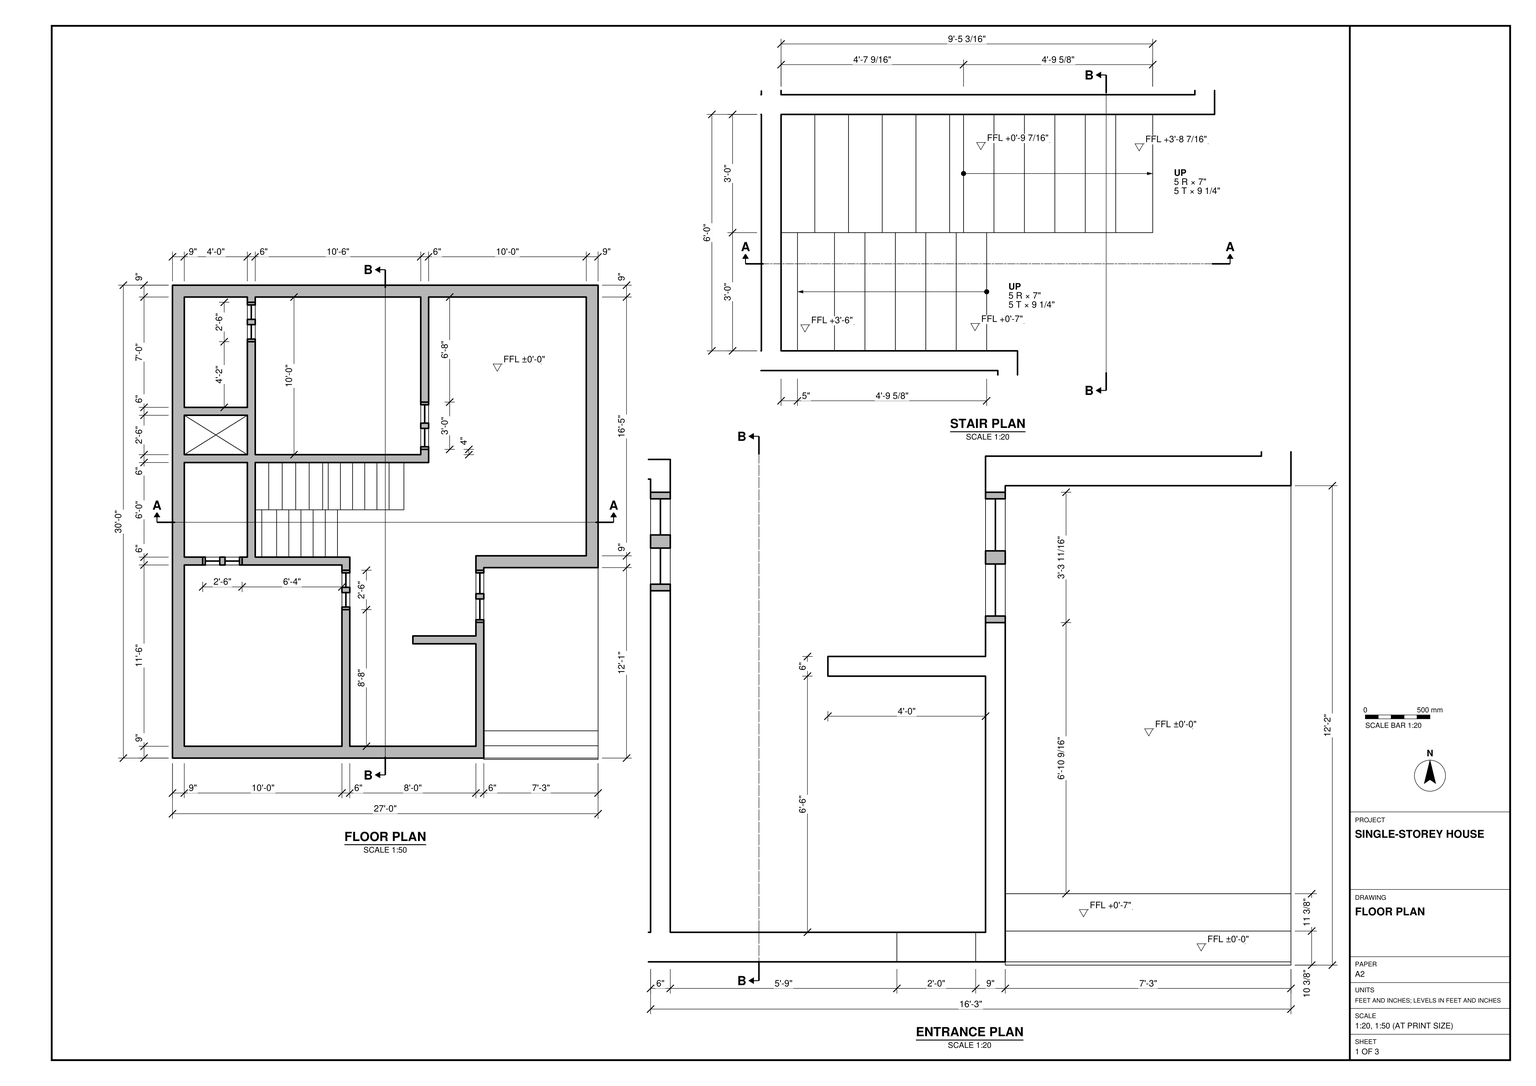
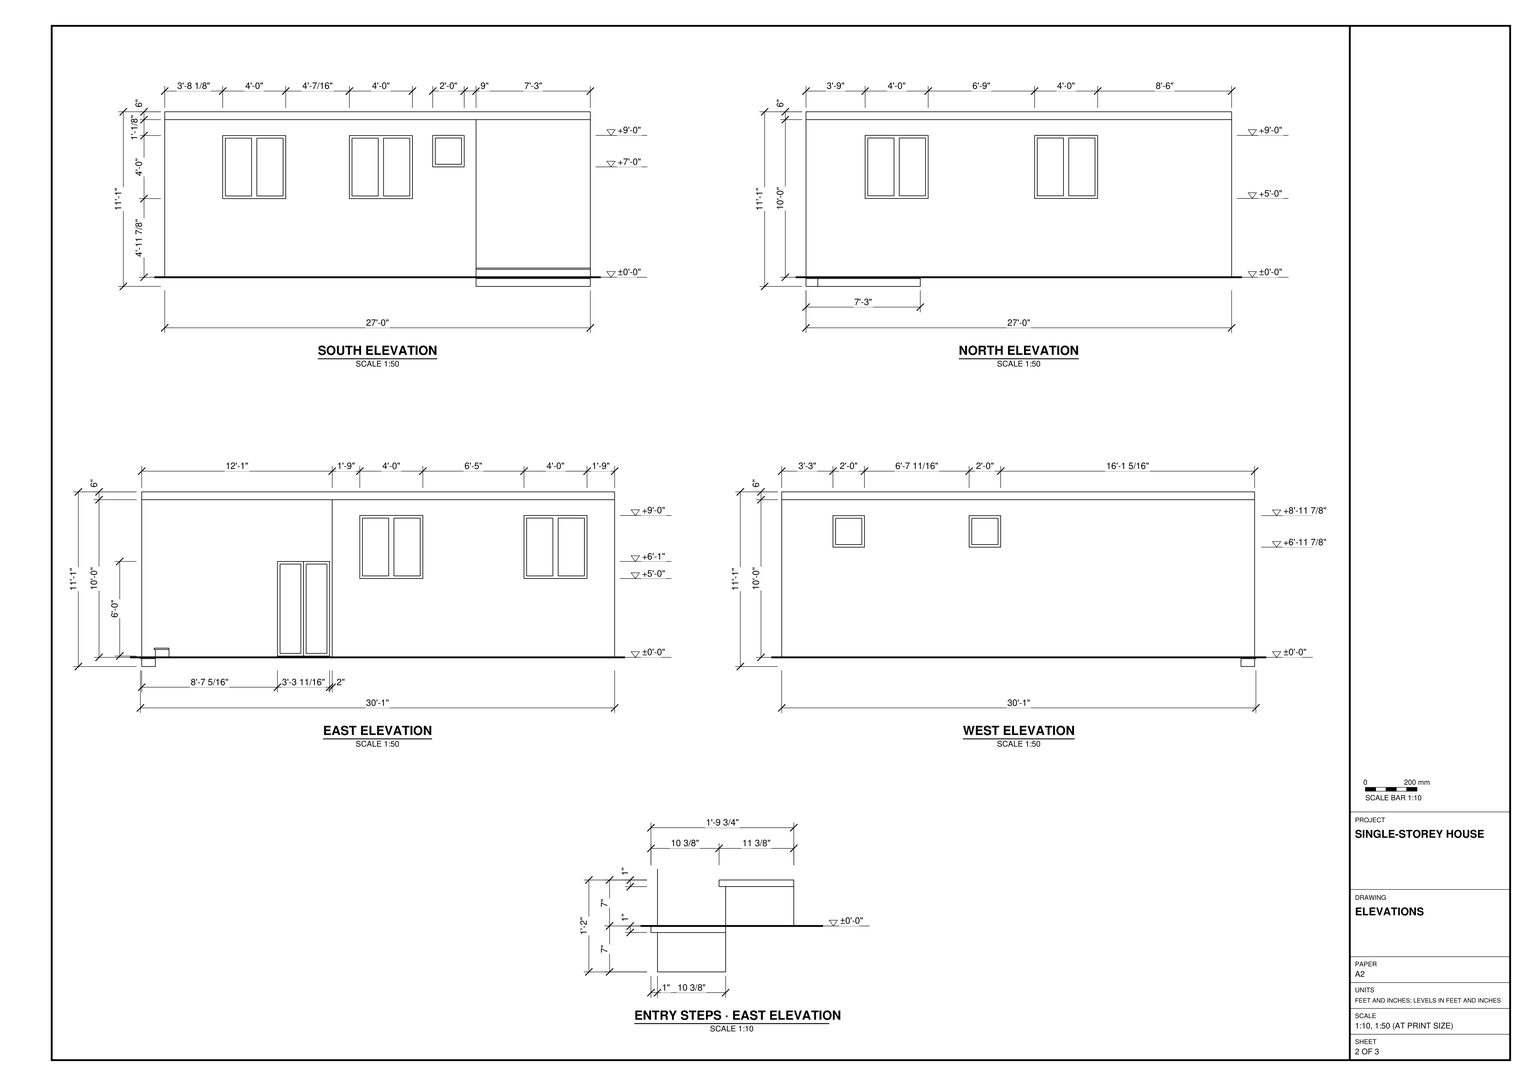
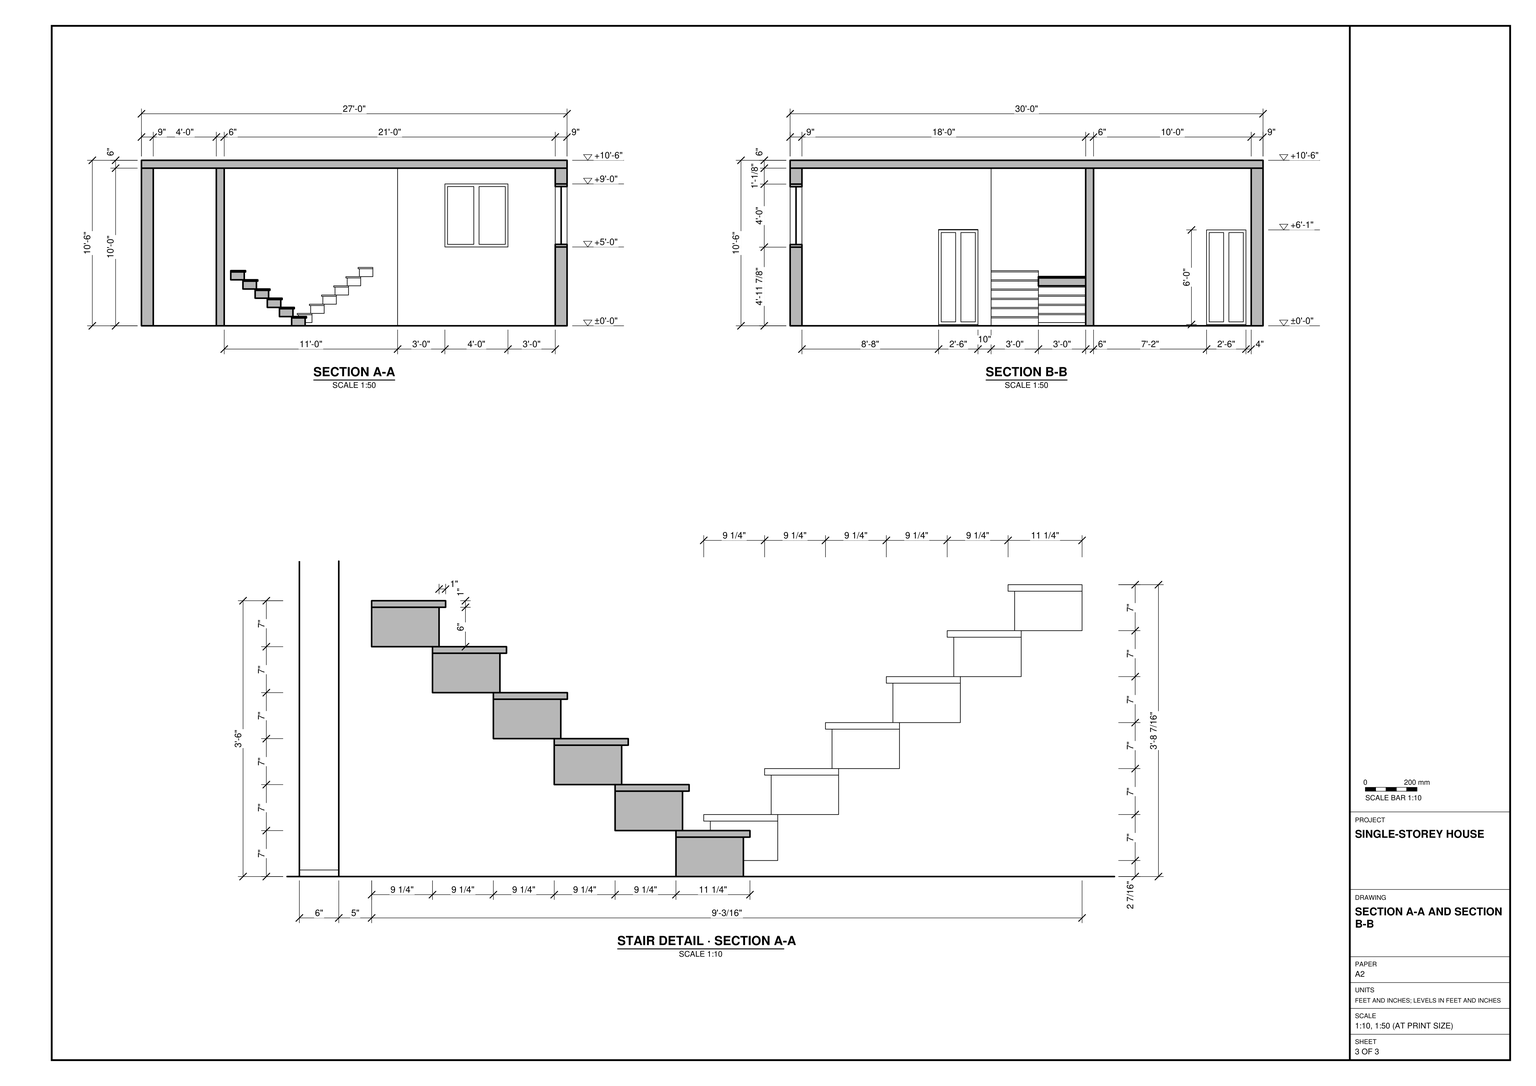
Build the house in SketchUp from task_files/diagram_01.pdf. Work in feet and inches, with the ground-floor finished level at ±0'-0". The overall dimensions are 27'-0" east to west, 30'-1" north to south and 11'-1" from the lowest part of the entry steps to the top of the roof.

Use the floor plan to set out the shell, including the recessed southeast entrance, the narrow rooms along the west side and the partitions around the central stair. Follow the drawn wall thicknesses, distinguishing the 9" exterior walls from the 6" partitions and returns where indicated. Model the floor and flat roof slab. Use the elevations to place the door and window openings and to distinguish the paired panes from the smaller square windows. Use the sections to set the window heights and the underside of the roof.

Model the entrance steps across the width of the recess. For the interior stair, use the stair plan for the position and direction of each flight and the enlarged section for the rises, tread spacing and projecting nosings. Decor and loose items, if used, may be any suitable library components. Keep walls, slabs, roof and any furniture or joinery pieces in separate groups or components, and use components for repeated parts. Save one SketchUp model as output_files/single_storey_house_with_recessed_entrance.skp.

# SketchUp Ruby script. Lengths in inches.
U = 1.inch
M = Sketchup.active_model
def pt(a) = Geom::Point3d.new(a.map { |v| v * U })
def face(e, loops, mat)
  f = e.add_face(loops[0].map { |a| pt(a) })
  loops[1..].each { |l| e.add_face(l.map { |a| pt(a) }).erase! }
  f.material = f.back_material = mat if mat
  f
end
# faces: each face lists its corners as indices into pts; further lists are holes
def faces(e, pts, list, mat = nil) = list.each { |f| face(e, (f[0].is_a?(Array) ? f : [f]).map { |l| l.map { |i| pts[i] } }, mat) }
# xy, xz, yz: faces in a plane at the given z, y or x. An outline is a flat list of corners, or four numbers for a rectangle; further outlines are holes
def ring(l) = l.size == 4 ? [[l[0], l[1]], [l[2], l[1]], [l[2], l[3]], [l[0], l[3]]] : l.each_slice(2).to_a
def flat(e, list, mat, &to3) = list.each { |f| face(e, (f[0].is_a?(Array) ? f : [f]).map { |l| ring(l).map { |u, v| to3.(u, v) } }, mat) }
def xy(e, z, list, mat = nil) = flat(e, list, mat) { |x, y| [x, y, z] }
def xz(e, y, list, mat = nil) = flat(e, list, mat) { |x, z| [x, y, z] }
def yz(e, x, list, mat = nil) = flat(e, list, mat) { |y, z| [x, y, z] }
def lines(e, pts, list) = list.each { |a, b| e.add_line(pt(pts[a]), pt(pts[b])) }
# prism: a flat outline (further loops are holes) pulled along v
def prism(e, loops, v, mat = nil)
  f = face(e, loops, mat); d = Geom::Vector3d.new(v.map { |x| x * U })
  f.pushpull(f.normal.samedirection?(d) ? d.length : -d.length)
end
def box(e, o, s, mat = nil) = prism(e, [[o, [o[0] + s[0], o[1], o[2]], [o[0] + s[0], o[1] + s[1], o[2]], [o[0], o[1] + s[1], o[2]]]], [0, 0, s[2]], mat)
def at(x, y, z, deg = 0) = Geom::Transformation.translation(pt([x, y, z])) * Geom::Transformation.rotation(ORIGIN, Z_AXIS, deg.degrees)
def axes(o, x, y, z) = Geom::Transformation.new([*x, 0, *y, 0, *z, 0, *pt(o).to_a, 1])
def part(name) = M.definitions.add(name)
# library, detail: a bought-in or finely detailed component or shape, given as its bounding box
def library(name, o, s) = part(name).tap { |d| box(d.entities, o, s) }
def detail(e, o, s) = box(e.add_group.entities, o, s)
def put(e, d, t, mat = nil) = e.add_instance(d, t).tap { |i| i.material = mat if mat }
def group(e, t, mat = nil) = e.add_group.tap { |g| g.transformation = t; g.material = mat if mat }.entities
root = M.entities
M.materials.add("[Checker Plate]").color = [245, 245, 245]
M.materials.add("[Granite Tile]").color = [155, 148, 143]
M.materials.add("[Tile Travertine 2 inch]").color = [181, 178, 172]
M.materials.add("[Translucent Glass Blue]").color = [100, 149, 237]
M.materials["[Translucent Glass Blue]"].alpha = 0.5
M.materials.add("[Translucent Glass Corrugated]").color = [141, 158, 145]
M.materials["[Translucent Glass Corrugated]"].alpha = 0.8
M.materials.add("[Wood Bamboo]").color = [177, 105, 43]
M.materials.add("[Wood Cherry Original]").color = [152, 86, 42]
M.materials.add("[Wood Veneer 02]").color = [190, 128, 91]
c1 = part("Group\#5")
xy(c1.entities,0,[[0,0,9,24],[0,24,9,48]])
xy(c1.entities,2,[[0,2,4.5,22],[4.5,2,9,22],[0,26,4.5,46],[4.5,26,9,46]],"[Wood Bamboo]")
xy(c1.entities,46,[[0,2,4.5,22],[4.5,2,9,22],[0,26,4.5,46],[4.5,26,9,46]],"[Wood Bamboo]")
xy(c1.entities,48,[[0,0,9,48]],"[Wood Bamboo]")
xz(c1.entities,0,[[0,0,9,48]],"[Wood Bamboo]")
xz(c1.entities,2,[[0,2,4.5,46],[4.5,2,9,46]],"[Wood Bamboo]")
xz(c1.entities,22,[[0,2,4.5,46],[4.5,2,9,46]],"[Wood Bamboo]")
xz(c1.entities,26,[[0,2,4.5,46],[4.5,2,9,46]],"[Wood Bamboo]")
xz(c1.entities,46,[[0,2,4.5,46],[4.5,2,9,46]],"[Wood Bamboo]")
xz(c1.entities,48,[[0,0,9,48]],"[Wood Bamboo]")
yz(c1.entities,0,[[[0,0,48,48],[2,2,22,46],[26,2,46,46]]],"[Wood Bamboo]")
yz(c1.entities,4.5,[[2,2,22,46],[26,2,46,46]],"[Translucent Glass Corrugated]")
yz(c1.entities,9,[[[0,0,48,48],[2,2,22,46],[26,2,46,46]]],"[Wood Bamboo]")
c2 = part("Group\#6")
xy(c2.entities,0,[[-9,0,0,24]],"[Wood Veneer 02]")
xy(c2.entities,2,[[-9,2,-4.5,22],[-4.5,2,0,22]],"[Wood Veneer 02]")
xy(c2.entities,22,[[-9,2,-4.5,22],[-4.5,2,0,22]],"[Wood Veneer 02]")
xy(c2.entities,24,[[-9,0,0,24]],"[Wood Veneer 02]")
xz(c2.entities,0,[[-9,0,0,24]],"[Wood Veneer 02]")
xz(c2.entities,2,[[-9,2,-4.5,22],[-4.5,2,0,22]],"[Wood Veneer 02]")
xz(c2.entities,22,[[-9,2,-4.5,22],[-4.5,2,0,22]],"[Wood Veneer 02]")
xz(c2.entities,24,[[-9,0,0,24]],"[Wood Veneer 02]")
yz(c2.entities,-9,[[[0,0,24,24],[2,2,22,22]]],"[Wood Veneer 02]")
yz(c2.entities,-4.5,[[2,2,22,22]],"[Checker Plate]")
yz(c2.entities,0,[[[0,0,24,24],[2,2,22,22]]],"[Wood Veneer 02]")
c3 = part("Group\#7")
xy(c3.entities,0,[[0,0,30,6]])
xy(c3.entities,1,[[0,0,30,6]],"[Tile Travertine 2 inch]")
xz(c3.entities,0,[[0,0,30,1]],"[Tile Travertine 2 inch]")
xz(c3.entities,6,[[0,0,30,1]],"[Tile Travertine 2 inch]")
yz(c3.entities,0,[[0,0,6,1]])
yz(c3.entities,30,[[0,0,6,1]])
c4 = part("Component\#1")
xz(c4.entities,0,[[0,0,11,68]])
c5 = part("Group\#8")
xy(c5.entities,0,[[0,-6,15,0],[15,-6,30,0]])
xy(c5.entities,2,[[2,-6,13,-3],[17,-6,28,0],[2,-3,13,0]],"[Wood Cherry Original]")
xy(c5.entities,70,[[2,-6,13,-3],[17,-6,28,0],[2,-3,13,0]],"[Wood Cherry Original]")
xy(c5.entities,72,[[0,-6,30,0]],"[Wood Cherry Original]")
xz(c5.entities,-6,[[[0,0,30,72],[2,2,13,70],[17,2,28,70]]],"[Wood Cherry Original]")
xz(c5.entities,0,[[[0,0,30,72],[2,2,13,70],[17,2,28,70]]],"[Wood Cherry Original]")
yz(c5.entities,0,[[-6,0,0,72]])
yz(c5.entities,2,[[-6,2,-3,70],[-3,2,0,70]],"[Wood Cherry Original]")
yz(c5.entities,13,[[-6,2,-3,70],[-3,2,0,70]],"[Wood Cherry Original]")
yz(c5.entities,17,[[-6,2,0,70]],"[Wood Cherry Original]")
yz(c5.entities,28,[[-6,2,0,70]],"[Wood Cherry Original]")
yz(c5.entities,30,[[-6,0,0,72]])
put(c5.entities,c4,at(2,-3,2),"[Wood Cherry Original]")
put(c5.entities,c4,at(17,-3,2),"[Wood Cherry Original]")
c6 = part("Group\#14")
xy(c6.entities,0,[[0,0,10.27,36]])
xz(c6.entities,0,[[0,0,10.27,6]])
xz(c6.entities,36,[[0,0,10.27,6]])
yz(c6.entities,0,[[0,0,36,6]])
yz(c6.entities,10.27,[[0,0,36,6]])
g1 = group(c6.entities,at(0,0,6))
box(g1,[0,0,0],[11.27,36,1])
xy(root,0,[[[0,1,204,1,204,10,135,10,135,114,129,114,129,10,9,10,9,148,23,148,23,154,9,154,9,226,57,226,57,154,53,154,53,148,129,148,129,144,135,144,135,154,63,154,63,226,195,226,195,236,189,236,189,232,63,232,63,318,57,318,57,268,9,268,9,352,57,352,57,348,63,348,63,352,189,352,189,272,195,272,195,352,315,352,315,155,231,155,231,144,237,144,237,146,324,146,324,361,0,361],[9,232,57,262]],[228,1,237,1,237,104.3,231,104.3,231,94,183,94,183,88,231,88,231,10,228,10],[237,1,324,11.375],[9,10,129,10,129,114,135,114,135,10,231,10,231,88,183,88,183,94,231,94,231,155,315,155,315,352,195,352,195,226,175.9375,226,175.9375,190,124.6,190,124.6,154,135,154,135,144,129,144,129,148,9,148],[237,21.75,324,146],
  [9,154,57,226],[63,154,73.27,190],[73.27,154,83.53,190],[83.53,154,93.8,190],[93.8,154,104.07,190],
  [104.07,154,114.34,190],[63,190,73.27,226],[73.27,190,83.53,226],[83.53,190,93.8,226],[93.8,190,104.07,226],
  [104.07,190,114.34,226],[114.34,190,124.6,226],[124.6,190,134.87,226],[134.87,190,145.14,226],[145.14,190,155.4,226],
  [155.4,190,165.67,226],[165.67,190,175.9375,226],[63,232,189,232,189,352,63,352,63,348,57,348,57,352,9,352,9,268,57,268,57,318,63,318],[9,232,33,247,9,262],[9,232,57,232,33,247],
  [57,232,57,262,33,247],[33,247,57,262,9,262]])
xy(root,59.875,[[44.125,1,92.125,10],[140.5625,1,188.5625,10]])
xy(root,60,[[315,167,324,215],[315,292,324,340],[102,352,150,361],[231,352,279,361]])
xy(root,73,[[231,104.3,237,144],[23,148,53,154],[189,236,195,272],[57,318,63,348]])
xy(root,83.875,[[0,194.3125,9,218.3125],[0,298,9,322]])
xy(root,84,[[204,1,228,10]])
xy(root,107.875,[[44.125,1,92.125,10],[140.5625,1,188.5625,10],[0,194.3125,9,218.3125],[0,298,9,322]])
xy(root,108,[[204,1,228,10],[315,167,324,215],[315,292,324,340],[102,352,150,361],[231,352,279,361]])
xy(root,120,[[[0,1,237,1,237,146,324,146,324,361,0,361],[135,10,135,154,63,154,63,226,195,226,195,352,315,352,315,155,231,155,231,94,183,94,183,88,231,88,231,10],[9,10,129,148],[63,232,189,352],[9,268,57,352],[9,154,57,226],[9,232,57,262]]])
xz(root,1,[[[0,0,237,120],[44.125,59.875,92.125,107.875],[140.5625,59.875,188.5625,107.875],[204,84,228,108]]])
xz(root,10,[[[9,0,129,120],[44.125,59.875,92.125,107.875]],[[135,0,231,120],[140.5625,59.875,188.5625,107.875],[204,84,228,108]]])
xz(root,88,[[183,0,231,120]])
xz(root,94,[[183,0,231,120]])
xz(root,104.3,[[231,0,237,73]])
xz(root,114,[[129,0,129,73,135,73.33,135,0]])
xz(root,144,[[129,0,135,0,135,73.33,129,73],[231,0,237,73]])
xz(root,146,[[237,0,324,120]])
xz(root,148,[[9,0,23,0,23,73,53,73,53,0,129,0,129,120,9,120]])
xz(root,154,[[9,0,9,120,57,120,57,0,53,0,53,73,23,73,23,0],[23,0,53,1],[63,0,135,120]])
xz(root,155,[[231,0,315,120]])
xz(root,167,[[315,60,324,108]])
xz(root,194.3125,[[0,83.875,9,107.875]])
xz(root,215,[[315,60,324,108]])
xz(root,218.3125,[[0,83.875,9,107.875]])
xz(root,226,[[9,0,57,120],[63,0,195,120]])
xz(root,232,[[9,0,57,120],[63,0,189,120]])
xz(root,236,[[189,0,195,73]])
xz(root,262,[[9,0,57,120]])
xz(root,268,[[9,0,57,120]])
xz(root,272,[[189,0,195,73]])
xz(root,292,[[315,60,324,108]])
xz(root,298,[[0,83.875,9,107.875]])
xz(root,318,[[57,0,63,73]])
xz(root,322,[[0,83.875,9,107.875]])
xz(root,340,[[315,60,324,108]])
xz(root,348,[[57,0,63,73]])
xz(root,352,[[9,0,57,120],[[63,0,189,120],[102,60,150,108]],[[195,0,315,120],[231,60,279,108]]])
xz(root,361,[[[0,0,324,120],[102,60,150,108],[231,60,279,108]]])
yz(root,0,[[[1,0,361,120],[194.3125,83.875,218.3125,107.875],[298,83.875,322,107.875]]])
yz(root,9,[[10,0,148,120],[[154,0,226,120],[194.3125,83.875,218.3125,107.875]],[232,0,262,120],[[268,0,352,120],[298,83.875,322,107.875]]])
yz(root,23,[[148,0,154,73]])
yz(root,44.125,[[1,59.875,10,107.875]])
yz(root,53,[[148,0,154,73]])
yz(root,57,[[154,0,226,120],[232,0,262,120],[268,0,268,120,352,120,352,0,348,0,348,73,318,73,318,0]])
yz(root,63,[[154,0,226,120],[232,0,318,0,318,73,348,73,348,0,352,0,352,120,232,120]])
yz(root,92.125,[[1,59.875,10,107.875]])
yz(root,102,[[352,60,361,108]])
yz(root,129,[[10,0,10,120,148,120,148,0,144,0,144,73,114,73,114,0]])
yz(root,135,[[10,0,114,0,114,73.33,144,73.33,144,0,154,0,154,120,10,120]])
yz(root,140.5625,[[1,59.875,10,107.875]])
yz(root,150,[[352,60,361,108]])
yz(root,183,[[88,0,94,120]])
yz(root,188.5625,[[1,59.875,10,107.875]])
yz(root,189,[[232,0,232,120,352,120,352,0,272,0,272,73,236,73,236,0]])
yz(root,195,[[226,0,236,0,236,73,272,73,272,0,352,0,352,120,226,120]])
yz(root,204,[[1,84,10,108]])
yz(root,228,[[1,84,10,108]])
yz(root,231,[[10,0,88,120],[94,0,94,120,155,120,155,0,144,0,144,73,103.7,73,103.7,1,104.3,1,104.3,0],[103.7,1,104.3,73],[352,60,361,108]])
yz(root,237,[[1,0,104.3,0,104.3,73,144,73,144,0,146,0,146,120,1,120]])
yz(root,279,[[352,60,361,108]])
yz(root,315,[[[155,0,352,120],[167,60,215,108],[292,60,340,108]]])
yz(root,324,[[[146,0,361,120],[167,60,215,108],[292,60,340,108]]])
p = [[135,114,73.33],[129,114,73],[129,144,73],[135,144,73.33]]
faces(root,p,[[0,1,2,3]])
g2 = group(root,at(237,11.375,0))
xy(g2,0,[[0,0,87,10.375]])
xz(g2,0,[[0,0,87,6]])
xz(g2,10.375,[[0,0,78,6],[78,0,87,6]])
yz(g2,0,[[0,0,10.375,6]])
yz(g2,87,[[0,0,10.375,6]])
g3 = group(g2,at(0,0,6))
prism(g3,[[[0,-1,0],[0,10.375,0],[78,10.375,0],[87,10.375,0],[87,-1,0]]],[0,0,1])
g4 = group(root,at(237,1,-7))
xy(g4,0,[[0,0,87,10.375]])
xz(g4,0,[[0,0,87,6]])
xz(g4,10.375,[[0,0,78,6],[78,0,87,6]])
yz(g4,0,[[0,0,10.375,6]])
yz(g4,87,[[0,0,10.375,6]])
g5 = group(g4,at(0,0,6))
prism(g5,[[[0,-1,0],[0,10.375,0],[78,10.375,0],[87,10.375,0],[87,-1,0]]],[0,0,1])
put(root,c1,at(315,167,60))
put(root,c1,at(315,292,60))
put(root,c1,at(279,352,60,90))
put(root,c1,at(92.125,1,59.875,90))
put(root,c1,at(188.5625,1,59.875,90))
put(root,c1,at(150,352,60,90))
put(root,c2,at(9,194.3125,83.875))
put(root,c2,at(9,298,83.875))
put(root,c3,at(23,148,0))
put(root,c5,at(23,154,1))
put(root,c5,at(129,114,1,90),"[Wood Cherry Original]")
put(root,c3,at(135,114,0,90))
g6 = group(root,at(231,104,0))
xy(g6,0,[[0,0.3,6,40]])
xy(g6,1,[[0,0.3,6,40]],"[Granite Tile]")
xz(g6,0.3,[[0,0,6,1]])
xz(g6,40,[[0,0,6,1]])
yz(g6,0,[[0.3,0,40,1]],"[Granite Tile]")
yz(g6,6,[[0.3,0,40,1]],"[Granite Tile]")
g7 = group(root,at(231,104.3,1))
xy(g7,0,[[0,0,6,19.85],[0,19.85,6,39.7]])
xy(g7,2,[[0,2,3,17.85],[3,2,6,17.85],[0,21.85,3,37.7],[3,21.85,6,37.7]],"[Wood Cherry Original]")
xy(g7,70,[[0,2,3,17.85],[3,2,6,17.85],[0,21.85,3,37.7],[3,21.85,6,37.7]],"[Wood Cherry Original]")
xy(g7,72,[[0,0,6,39.7]],"[Wood Cherry Original]")
xz(g7,0,[[0,0,6,72]])
xz(g7,2,[[0,2,3,70],[3,2,6,70]],"[Wood Cherry Original]")
xz(g7,17.85,[[0,2,3,70],[3,2,6,70]],"[Wood Cherry Original]")
xz(g7,21.85,[[0,2,3,70],[3,2,6,70]],"[Wood Cherry Original]")
xz(g7,37.7,[[0,2,3,70],[3,2,6,70]],"[Wood Cherry Original]")
xz(g7,39.7,[[0,0,6,72]])
yz(g7,0,[[[0,0,39.7,72],[21.85,2,37.7,70],[2,2,17.85,70]]],"[Wood Cherry Original]")
yz(g7,3,[[2,2,17.85,70],[21.85,2,37.7,70]],"[Wood Cherry Original]")
yz(g7,6,[[[0,0,19.85,72],[2,2,17.85,70]],[[19.85,0,39.7,72],[21.85,2,37.7,70]]],"[Wood Cherry Original]")
p = [[6,39.7,72],[6,40,72]]
lines(g7,p,[[0,1]])
g8 = group(root,at(189,236,0))
xy(g8,0,[[0,0,6,36]])
xy(g8,1,[[0,0,6,36]],"[Granite Tile]")
xz(g8,0,[[0,0,6,1]])
xz(g8,36,[[0,0,6,1]])
yz(g8,0,[[0,0,36,1]],"[Granite Tile]")
yz(g8,6,[[0,0,36,1]],"[Granite Tile]")
g9 = group(root,at(189,236,73))
xy(g9,-72,[[0,0,6,18],[0,18,6,36]])
xy(g9,-70,[[0,2,3,16],[3,2,6,16],[0,20,3,34],[3,20,6,34]],"[Wood Cherry Original]")
xy(g9,-2,[[0,2,3,16],[3,2,6,16],[0,20,3,34],[3,20,6,34]])
xy(g9,0,[[0,0,6,36]],"[Wood Cherry Original]")
xz(g9,0,[[0,-72,6,0]])
xz(g9,2,[[0,-70,3,-2],[3,-70,6,-2]],"[Wood Cherry Original]")
xz(g9,16,[[0,-70,3,-2],[3,-70,6,-2]],"[Wood Cherry Original]")
xz(g9,20,[[0,-70,3,-2],[3,-70,6,-2]],"[Wood Cherry Original]")
xz(g9,34,[[0,-70,3,-2],[3,-70,6,-2]],"[Wood Cherry Original]")
xz(g9,36,[[0,-72,6,0]])
yz(g9,0,[[[0,-72,36,0],[2,-70,16,-2],[20,-70,34,-2]]],"[Wood Cherry Original]")
yz(g9,3,[[2,-70,16,-2],[20,-70,34,-2]],"[Wood Cherry Original]")
yz(g9,6,[[[0,-72,18,0],[2,-70,16,-2]],[[18,-72,36,0],[20,-70,34,-2]]],"[Wood Cherry Original]")
put(root,c5,at(57,318,1,90),"[Wood Cherry Original]")
put(root,c3,at(63,318,0,90))
g10 = group(root,at(204,10,84))
xy(g10,0,[[0,-9,24,0]])
xy(g10,2,[[2,-9,22,-4.5],[2,-4.5,22,0]],"[Wood Cherry Original]")
xy(g10,22,[[2,-9,22,-4.5],[2,-4.5,22,0]],"[Wood Cherry Original]")
xy(g10,24,[[0,-9,24,0]],"[Wood Cherry Original]")
xz(g10,-9,[[[0,0,24,24],[2,2,22,22]]],"[Wood Cherry Original]")
xz(g10,-4.5,[[2,2,22,22]],"[Translucent Glass Blue]")
xz(g10,0,[[[0,0,24,24],[2,2,22,22]]],"[Wood Cherry Original]")
yz(g10,0,[[-9,0,0,24]],"[Wood Cherry Original]")
yz(g10,2,[[-9,2,-4.5,22],[-4.5,2,0,22]],"[Wood Cherry Original]")
yz(g10,22,[[-9,2,-4.5,22],[-4.5,2,0,22]],"[Wood Cherry Original]")
yz(g10,24,[[-9,0,0,24]],"[Wood Cherry Original]")
put(root,c6,at(114.34,154,0))
put(root,c6,at(105.07,154,7))
put(root,c6,at(95.8,154,14))
put(root,c6,at(86.53,154,21))
put(root,c6,at(77.27,154,28))
put(root,c6,at(68,154,35))
put(root,c6,at(139.1,226,9.44,180))
put(root,c6,at(148.36,226,16.44,180))
put(root,c6,at(157.63,226,23.44,180))
put(root,c6,at(176.17,226,37.44,180))
put(root,c6,at(129.83,226,2.44,180))
put(root,c6,at(166.9,226,30.44,180))
g11 = group(root,at(0,1,120))
box(g11,[0,0,0],[324,360,6])
